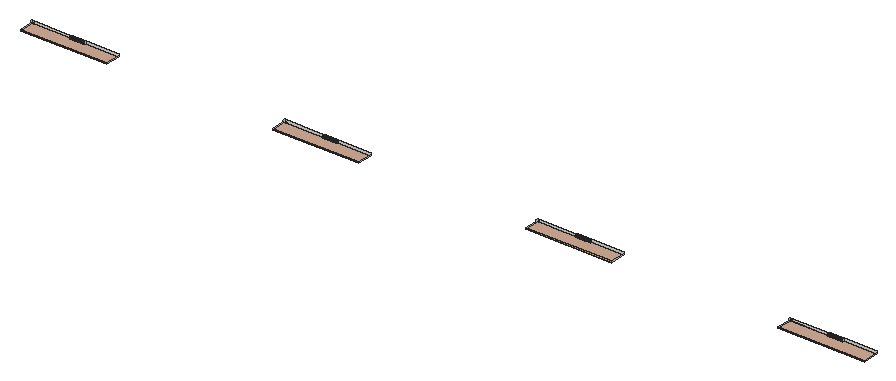
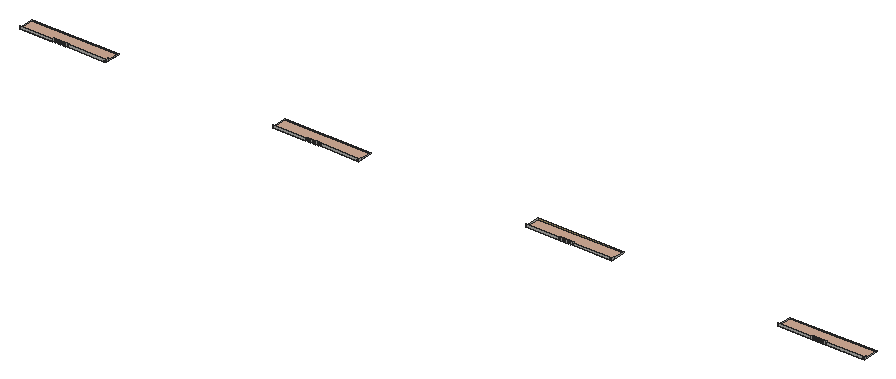
# SketchUp Ruby script. Lengths in inches.
U = 1.inch
M = Sketchup.active_model
def pt(a) = Geom::Point3d.new(a.map { |v| v * U })
def face(e, loops, mat)
  f = e.add_face(loops[0].map { |a| pt(a) })
  loops[1..].each { |l| e.add_face(l.map { |a| pt(a) }).erase! }
  f.material = f.back_material = mat if mat
  f
end
# faces: each face lists its corners as indices into pts; further lists are holes
def faces(e, pts, list, mat = nil) = list.each { |f| face(e, (f[0].is_a?(Array) ? f : [f]).map { |l| l.map { |i| pts[i] } }, mat) }
# xy, xz, yz: faces in a plane at the given z, y or x. An outline is a flat list of corners, or four numbers for a rectangle; further outlines are holes
def ring(l) = l.size == 4 ? [[l[0], l[1]], [l[2], l[1]], [l[2], l[3]], [l[0], l[3]]] : l.each_slice(2).to_a
def flat(e, list, mat, &to3) = list.each { |f| face(e, (f[0].is_a?(Array) ? f : [f]).map { |l| ring(l).map { |u, v| to3.(u, v) } }, mat) }
def xy(e, z, list, mat = nil) = flat(e, list, mat) { |x, y| [x, y, z] }
def xz(e, y, list, mat = nil) = flat(e, list, mat) { |x, z| [x, y, z] }
def yz(e, x, list, mat = nil) = flat(e, list, mat) { |y, z| [x, y, z] }
def lines(e, pts, list) = list.each { |a, b| e.add_line(pt(pts[a]), pt(pts[b])) }
# prism: a flat outline (further loops are holes) pulled along v
def prism(e, loops, v, mat = nil)
  f = face(e, loops, mat); d = Geom::Vector3d.new(v.map { |x| x * U })
  f.pushpull(f.normal.samedirection?(d) ? d.length : -d.length)
end
def box(e, o, s, mat = nil) = prism(e, [[o, [o[0] + s[0], o[1], o[2]], [o[0] + s[0], o[1] + s[1], o[2]], [o[0], o[1] + s[1], o[2]]]], [0, 0, s[2]], mat)
def at(x, y, z, deg = 0) = Geom::Transformation.translation(pt([x, y, z])) * Geom::Transformation.rotation(ORIGIN, Z_AXIS, deg.degrees)
def axes(o, x, y, z) = Geom::Transformation.new([*x, 0, *y, 0, *z, 0, *pt(o).to_a, 1])
def part(name) = M.definitions.add(name)
# library, detail: a bought-in or finely detailed component or shape, given as its bounding box
def library(name, o, s) = part(name).tap { |d| box(d.entities, o, s) }
def detail(e, o, s) = box(e.add_group.entities, o, s)
def put(e, d, t, mat = nil) = e.add_instance(d, t).tap { |i| i.material = mat if mat }
def group(e, t, mat = nil) = e.add_group.tap { |g| g.transformation = t; g.material = mat if mat }.entities
root = M.entities
M.materials.add("[Granite Brown]").color = [209, 172, 151]
M.materials.add("[Stone Brushed Khaki]").color = [226, 197, 133]
xy(root,771.4375,[[551.76,576.96,551.76,651.03,742.44,651.03,742.44,647.91,751.56,647.91,751.56,651.03,755.44,651.03,755.44,647.91,764.56,647.91,764.56,651.03,768.19,651.03,768.19,648.85,777.31,648.85,777.31,651.03,780.32,651.03,780.32,648.85,789.43,648.85,789.43,651.03,792.69,651.03,792.69,648.85,801.81,648.85,801.81,651.03,805.57,651.03,805.57,648.85,814.68,648.85,814.68,651.03,977.59,651.03,977.59,576.96],[1802.38,576.96,1802.38,651.03,1993.07,651.03,1993.07,647.91,2002.18,647.91,2002.18,651.03,2006.07,651.03,2006.07,647.91,2015.18,647.91,2015.18,651.03,2018.82,651.03,2018.82,648.85,2027.93,648.85,2027.93,651.03,2030.94,651.03,2030.94,648.85,2040.06,648.85,2040.06,651.03,2043.32,651.03,2043.32,648.85,2052.43,648.85,2052.43,651.03,2056.19,651.03,2056.19,648.85,2065.31,648.85,2065.31,651.03,2228.22,651.03,2228.22,576.96],[3053.01,576.96,3053.01,651.03,3243.69,651.03,3243.69,647.91,3252.81,647.91,3252.81,651.03,3256.69,651.03,3256.69,647.91,3265.81,647.91,3265.81,651.03,3269.44,651.03,3269.44,648.85,3278.56,648.85,3278.56,651.03,3281.57,651.03,3281.57,648.85,3290.68,648.85,3290.68,651.03,3293.94,651.03,3293.94,648.85,3303.06,648.85,3303.06,651.03,3306.82,651.03,3306.82,648.85,3315.93,648.85,3315.93,651.03,3478.84,651.03,3478.84,576.96],[4303.63,576.96,4303.63,651.03,4494.32,651.03,4494.32,647.91,4503.43,647.91,4503.43,651.03,4507.32,651.03,4507.32,647.91,4516.43,647.91,4516.43,651.03,4520.07,651.03,4520.07,648.85,4529.18,648.85,4529.18,651.03,4532.19,651.03,4532.19,648.85,4541.31,648.85,4541.31,651.03,4544.57,651.03,4544.57,648.85,4553.68,648.85,4553.68,651.03,4557.44,651.03,4557.44,648.85,4566.56,648.85,4566.56,651.03,4729.47,651.03,4729.47,576.96]],"[Granite Brown]")
xz(root,576.96,[[551.76,771.4375,977.59,776.0625],[1802.38,771.4375,2228.22,776.0625],[3053.01,771.4375,3478.84,776.0625],[4303.63,771.4375,4729.47,776.0625]],"[Stone Brushed Khaki]")
xz(root,647.91,[[742.44,771.4375,751.56,784.4375],[755.44,771.4375,764.56,784.4375],[1993.07,771.4375,2002.18,784.4375],[2006.07,771.4375,2015.18,784.4375],[3243.69,771.4375,3252.81,784.4375],
  [3256.69,771.4375,3265.81,784.4375],[4494.32,771.4375,4503.43,784.4375],[4507.32,771.4375,4516.43,784.4375]])
xz(root,648.85,[[768.19,771.4375,777.31,784.4375],[780.32,771.4375,789.43,784.4375],[792.69,771.4375,801.81,784.4375],[805.57,771.4375,814.68,784.4375],[2018.82,771.4375,2027.93,784.4375],
  [2030.94,771.4375,2040.06,784.4375],[2043.32,771.4375,2052.43,784.4375],[2056.19,771.4375,2065.31,784.4375],[3269.44,771.4375,3278.56,784.4375],[3281.57,771.4375,3290.68,784.4375],
  [3293.94,771.4375,3303.06,784.4375],[3306.82,771.4375,3315.93,784.4375],[4520.07,771.4375,4529.18,784.4375],[4532.19,771.4375,4541.31,784.4375],[4544.57,771.4375,4553.68,784.4375],
  [4557.44,771.4375,4566.56,784.4375]])
xz(root,651.03,[[551.76,771.4375,563.08,772.4375],[563.08,771.4375,563.08,778.4375,551.76,778.4375,551.76,784.4375,742.44,784.4375,742.44,771.4375],[751.56,771.4375,755.44,784.4375],[764.56,771.4375,768.19,784.4375],[777.31,771.4375,780.32,784.4375],
  [789.43,771.4375,792.69,784.4375],[801.81,771.4375,805.57,784.4375],[814.68,771.4375,814.89,772.4375],[814.89,771.4375,814.89,772.4375,814.68,772.4375,814.68,784.4375,977.59,784.4375,977.59,771.4375],[1802.38,771.4375,1813.71,772.4375],
  [1813.71,771.4375,1813.71,778.4375,1802.38,778.4375,1802.38,784.4375,1993.07,784.4375,1993.07,771.4375],[2002.18,771.4375,2006.07,784.4375],[2015.18,771.4375,2018.82,784.4375],[2027.93,771.4375,2030.94,784.4375],[2040.06,771.4375,2043.32,784.4375],
  [2052.43,771.4375,2056.19,784.4375],[2065.31,771.4375,2065.52,772.4375],[2065.52,771.4375,2065.52,772.4375,2065.31,772.4375,2065.31,784.4375,2228.22,784.4375,2228.22,771.4375],[3053.01,771.4375,3064.33,772.4375],[3064.33,771.4375,3064.33,778.4375,3053.01,778.4375,3053.01,784.4375,3243.69,784.4375,3243.69,771.4375],
  [3252.81,771.4375,3256.69,784.4375],[3265.81,771.4375,3269.44,784.4375],[3278.56,771.4375,3281.57,784.4375],[3290.68,771.4375,3293.94,784.4375],[3303.06,771.4375,3306.82,784.4375],
  [3315.93,771.4375,3316.14,772.4375],[3316.14,771.4375,3316.14,772.4375,3315.93,772.4375,3315.93,784.4375,3478.84,784.4375,3478.84,771.4375],[4303.63,771.4375,4314.96,772.4375],[4314.96,771.4375,4314.96,778.4375,4303.63,778.4375,4303.63,784.4375,4494.32,784.4375,4494.32,771.4375],[4503.43,771.4375,4507.32,784.4375],
  [4516.43,771.4375,4520.07,784.4375],[4529.18,771.4375,4532.19,784.4375],[4541.31,771.4375,4544.57,784.4375],[4553.68,771.4375,4557.44,784.4375],[4566.56,771.4375,4566.77,772.4375],
  [4566.77,771.4375,4566.77,772.4375,4566.56,772.4375,4566.56,784.4375,4729.47,784.4375,4729.47,771.4375]])
yz(root,551.76,[[576.96,771.4375,640.11,776.0625],[640.11,771.4375,651.03,784.4375]])
yz(root,742.44,[[647.91,771.4375,651.03,784.4375]])
yz(root,751.56,[[647.91,771.4375,651.03,784.4375]])
yz(root,755.44,[[647.91,771.4375,651.03,784.4375]])
yz(root,764.56,[[647.91,771.4375,651.03,784.4375]])
yz(root,768.19,[[648.85,771.4375,651.03,784.4375]])
yz(root,777.31,[[648.85,771.4375,651.03,784.4375]])
yz(root,780.32,[[648.85,771.4375,651.03,784.4375]])
yz(root,789.43,[[648.85,771.4375,651.03,784.4375]])
yz(root,792.69,[[648.85,771.4375,651.03,784.4375]])
yz(root,801.81,[[648.85,771.4375,651.03,784.4375]])
yz(root,805.57,[[648.85,771.4375,651.03,784.4375]])
yz(root,814.68,[[648.85,771.4375,651.03,784.4375]])
yz(root,977.59,[[576.96,771.4375,651.03,776.0625]])
yz(root,1802.38,[[576.96,771.4375,640.11,776.0625],[640.11,771.4375,651.03,784.4375]])
yz(root,1993.07,[[647.91,771.4375,651.03,784.4375]])
yz(root,2002.18,[[647.91,771.4375,651.03,784.4375]])
yz(root,2006.07,[[647.91,771.4375,651.03,784.4375]])
yz(root,2015.18,[[647.91,771.4375,651.03,784.4375]])
yz(root,2018.82,[[648.85,771.4375,651.03,784.4375]])
yz(root,2027.93,[[648.85,771.4375,651.03,784.4375]])
yz(root,2030.94,[[648.85,771.4375,651.03,784.4375]])
yz(root,2040.06,[[648.85,771.4375,651.03,784.4375]])
yz(root,2043.32,[[648.85,771.4375,651.03,784.4375]])
yz(root,2052.43,[[648.85,771.4375,651.03,784.4375]])
yz(root,2056.19,[[648.85,771.4375,651.03,784.4375]])
yz(root,2065.31,[[648.85,771.4375,651.03,784.4375]])
yz(root,2228.22,[[576.96,771.4375,651.03,776.0625]])
yz(root,3053.01,[[576.96,771.4375,640.11,776.0625],[640.11,771.4375,651.03,784.4375]])
yz(root,3243.69,[[647.91,771.4375,651.03,784.4375]])
yz(root,3252.81,[[647.91,771.4375,651.03,784.4375]])
yz(root,3256.69,[[647.91,771.4375,651.03,784.4375]])
yz(root,3265.81,[[647.91,771.4375,651.03,784.4375]])
yz(root,3269.44,[[648.85,771.4375,651.03,784.4375]])
yz(root,3278.56,[[648.85,771.4375,651.03,784.4375]])
yz(root,3281.57,[[648.85,771.4375,651.03,784.4375]])
yz(root,3290.68,[[648.85,771.4375,651.03,784.4375]])
yz(root,3293.94,[[648.85,771.4375,651.03,784.4375]])
yz(root,3303.06,[[648.85,771.4375,651.03,784.4375]])
yz(root,3306.82,[[648.85,771.4375,651.03,784.4375]])
yz(root,3315.93,[[648.85,771.4375,651.03,784.4375]])
yz(root,3478.84,[[576.96,771.4375,651.03,776.0625]])
yz(root,4303.63,[[576.96,771.4375,640.11,776.0625],[640.11,771.4375,651.03,784.4375]])
yz(root,4494.32,[[647.91,771.4375,651.03,784.4375]])
yz(root,4503.43,[[647.91,771.4375,651.03,784.4375]])
yz(root,4507.32,[[647.91,771.4375,651.03,784.4375]])
yz(root,4516.43,[[647.91,771.4375,651.03,784.4375]])
yz(root,4520.07,[[648.85,771.4375,651.03,784.4375]])
yz(root,4529.18,[[648.85,771.4375,651.03,784.4375]])
yz(root,4532.19,[[648.85,771.4375,651.03,784.4375]])
yz(root,4541.31,[[648.85,771.4375,651.03,784.4375]])
yz(root,4544.57,[[648.85,771.4375,651.03,784.4375]])
yz(root,4553.68,[[648.85,771.4375,651.03,784.4375]])
yz(root,4557.44,[[648.85,771.4375,651.03,784.4375]])
yz(root,4566.56,[[648.85,771.4375,651.03,784.4375]])
yz(root,4729.47,[[576.96,771.4375,651.03,776.0625]])
